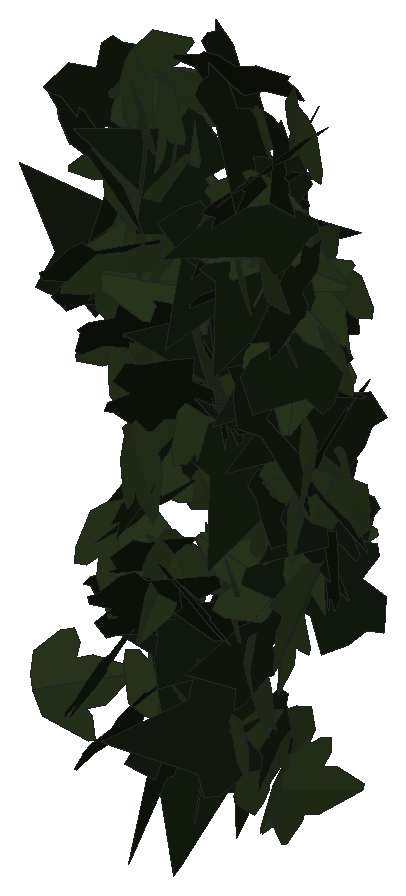
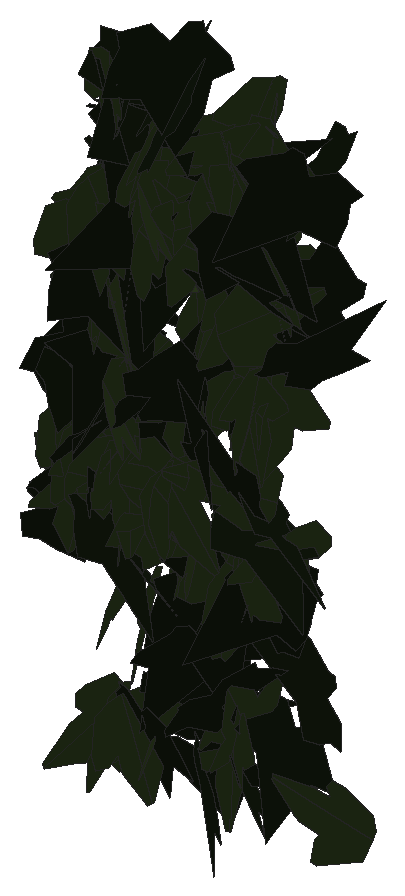
# SketchUp Ruby script. Lengths in inches.
U = 1.inch
M = Sketchup.active_model
def pt(a) = Geom::Point3d.new(a.map { |v| v * U })
def face(e, loops, mat)
  f = e.add_face(loops[0].map { |a| pt(a) })
  loops[1..].each { |l| e.add_face(l.map { |a| pt(a) }).erase! }
  f.material = f.back_material = mat if mat
  f
end
# faces: each face lists its corners as indices into pts; further lists are holes
def faces(e, pts, list, mat = nil) = list.each { |f| face(e, (f[0].is_a?(Array) ? f : [f]).map { |l| l.map { |i| pts[i] } }, mat) }
# xy, xz, yz: faces in a plane at the given z, y or x. An outline is a flat list of corners, or four numbers for a rectangle; further outlines are holes
def ring(l) = l.size == 4 ? [[l[0], l[1]], [l[2], l[1]], [l[2], l[3]], [l[0], l[3]]] : l.each_slice(2).to_a
def flat(e, list, mat, &to3) = list.each { |f| face(e, (f[0].is_a?(Array) ? f : [f]).map { |l| ring(l).map { |u, v| to3.(u, v) } }, mat) }
def xy(e, z, list, mat = nil) = flat(e, list, mat) { |x, y| [x, y, z] }
def xz(e, y, list, mat = nil) = flat(e, list, mat) { |x, z| [x, y, z] }
def yz(e, x, list, mat = nil) = flat(e, list, mat) { |y, z| [x, y, z] }
def lines(e, pts, list) = list.each { |a, b| e.add_line(pt(pts[a]), pt(pts[b])) }
# prism: a flat outline (further loops are holes) pulled along v
def prism(e, loops, v, mat = nil)
  f = face(e, loops, mat); d = Geom::Vector3d.new(v.map { |x| x * U })
  f.pushpull(f.normal.samedirection?(d) ? d.length : -d.length)
end
def box(e, o, s, mat = nil) = prism(e, [[o, [o[0] + s[0], o[1], o[2]], [o[0] + s[0], o[1] + s[1], o[2]], [o[0], o[1] + s[1], o[2]]]], [0, 0, s[2]], mat)
def at(x, y, z, deg = 0) = Geom::Transformation.translation(pt([x, y, z])) * Geom::Transformation.rotation(ORIGIN, Z_AXIS, deg.degrees)
def axes(o, x, y, z) = Geom::Transformation.new([*x, 0, *y, 0, *z, 0, *pt(o).to_a, 1])
def part(name) = M.definitions.add(name)
# library, detail: a bought-in or finely detailed component or shape, given as its bounding box
def library(name, o, s) = part(name).tap { |d| box(d.entities, o, s) }
def detail(e, o, s) = box(e.add_group.entities, o, s)
def put(e, d, t, mat = nil) = e.add_instance(d, t).tap { |i| i.material = mat if mat }
def group(e, t, mat = nil) = e.add_group.tap { |g| g.transformation = t; g.material = mat if mat }.entities
root = M.entities
M.materials.add("efeu1").color = [18, 25, 13]
M.materials.add("efeu2").color = [43, 57, 29]
c1 = part("ivyleaf_10")
p = [[0,0.5,-0.03],[-0.0625,2.02,-0.43],[-0.19,2.01,-0.46],[-0.54,1.05,-0.29],[-0.52,0.625,-0.18],[-0.83,0.76,-0.28],
  [-1.16,0.64,-0.33],[-1.15,0.33,-0.24],[-0.77,-0.39,0.02],[-0.3,-0.51,0.16],[0.04,-0.48,0.23],[-0.02,2.01,-0.4375],
  [-0.06,2.01,-0.43],[0.04,-0.49,0.23],[0.67,-0.49,0.14],[1.38,0.36,-0.2],[1.375,0.51,-0.24],[0.81,0.65,-0.19],
  [0.62,0.59,-0.15],[0.6,1.09,-0.28],[0.5,1.23,-0.31]]
faces(c1.entities,p,[[0,1,2,3,4,5,6,7,8,9,10],[11,12,0,13,14,15,16,17,18,19,20]],"efeu2")
c2 = part("ivyleaf_9")
p = [[1.54,2.16,1.25],[1.36,2.04,1.19],[-0.21,0.99,0.68],[-0.71,1.11,0.82],[-0.85,0.86,0.67],[-0.8,0.17,0.21],
  [-0.9,-0.01,0.1],[-0.67,-0.16,-0.02],[-0.08,-0.08,-0.05],[-0.03,-0.6,-0.4],[0.65,-0.88,-0.66],[0.83,-0.6,-0.49],
  [1.29,-0.42,-0.43],[1.8125,-0.07,-0.26],[1.21,0.44,0.15]]
faces(c2.entities,p,[[0,1,2,3,4,5,6,7,8,9,10,11,12,13,14]],"efeu1")
put(root,c1,axes([51.53,222.47,218.5625],[-0.09013,0.46947,0.14655],[-0.095,0.12957,-0.47348],[-0.48255,-0.11319,0.06584]))
put(root,c2,axes([50.85,222.37,215.3],[-0.1452,0.47845,-0.00029],[-0.00094,0.00002,0.5],[0.47845,0.1452,0.0009]))
put(root,c2,axes([51.6,222.35,219.3125],[0.35261,0.16273,0.31494],[0.29339,0.11538,-0.38809],[-0.19898,0.45848,-0.01412]))
put(root,c2,axes([53.29,222.89,221.95],[-0.4713,-0.01796,0.166],[-0.152,-0.15955,-0.44882],[0.06909,-0.47352,0.14493]))
put(root,c2,axes([53.6,222.66,221.11],[-0.40142,0.29572,0.03759],[-0.03003,0.02261,-0.49859],[-0.29659,-0.40254,-0.00039]))
put(root,c1,axes([53.06,222.78,221.97],[0.37689,0.10748,-0.31049],[-0.3067,-0.05441,-0.39112],[-0.11786,0.48527,0.02491]))
put(root,c1,axes([51.17,222.7,220.59],[-0.27641,-0.41637,-0.01513],[0.00782,0.01297,-0.49977],[0.41657,-0.27652,-0.00066]))
put(root,c2,axes([50.44,222.85,222.03],[0.31276,-0.37154,0.1189],[0.08783,-0.08142,-0.48544],[0.38009,0.32454,0.01433]))
put(root,c2,axes([53,222.84,222.1],[-0.1065,0.34539,-0.34549],[0.01072,-0.35187,-0.35507],[-0.48841,-0.08304,0.06754]))
put(root,c1,axes([51.28,222.55,220.52],[0.32321,-0.38109,-0.01756],[0.38148,0.32305,0.01069],[0.0032,-0.02031,0.49958]))
put(root,c2,axes([52.9,223.02,221.21],[-0.35666,-0.34673,-0.05072],[0.0462,0.02521,-0.49722],[0.34736,-0.35937,0.01405]))
put(root,c1,axes([51.41,222.7,222.22],[0.2972,-0.3609,-0.17726],[-0.02517,0.20329,-0.45611],[0.4013,0.28004,0.10267]))
put(root,c1,axes([51.01,222.82,217.28],[0.21033,0.447,-0.07716],[-0.03053,-0.0709,-0.494],[-0.45258,0.21252,-0.00253]))
put(root,c2,axes([51.21,222.53,216.45],[0.19094,0.36808,-0.27939],[0.12822,0.24824,0.41465],[0.44396,-0.22999,0.00041]))
put(root,c2,axes([50.56,222.55,220.26],[0.20508,0.39106,-0.23455],[0.09026,0.21728,0.44118],[0.44699,-0.22329,0.01853]))
put(root,c1,axes([53.11,222.69,221.28],[-0.39687,0.26741,0.14488],[-0.13605,0.05692,-0.47775],[-0.27201,-0.41863,0.02758]))
put(root,c1,axes([51.57,223.06,216.97],[0.04111,0.35247,-0.35225],[-0.05375,-0.34824,-0.35474],[-0.4954,0.06703,0.00926]))
put(root,c2,axes([52.31,223.21,222.66],[0.07999,-0.40668,0.27966],[0.05668,-0.27387,-0.41447],[0.4903,0.09801,0.00229]))
put(root,c1,axes([53.36,223.11,217.25],[0.11599,-0.43936,0.20859],[0.05478,-0.20127,-0.45441],[0.48326,0.12827,0.00144]))
put(root,c2,axes([52.375,223.15,215.03],[-0.2948,-0.08589,0.39461],[-0.37797,-0.11338,-0.30705],[0.14223,-0.47934,0.00192]))
put(root,c2,axes([51.16,222.59,219.98],[0.24192,0.42964,0.083],[0.04242,0.07137,-0.49306],[-0.43552,0.2456,-0.00191]))
put(root,c2,axes([52.2,223.27,221.01],[-0.19816,-0.42517,0.1731],[-0.07988,-0.15373,-0.46903],[0.45205,-0.21354,-0.007]))
put(root,c1,axes([51.1,222.91,221.77],[-0.42511,-0.26303,0.00996],[-0.00843,-0.00531,-0.4999],[0.26309,-0.42519,0.00008]))
put(root,c2,axes([51.81,223.1875,221.69],[-0.2757,-0.30734,-0.28201],[-0.07306,-0.29724,0.39536],[-0.41067,0.25921,0.11899]))
put(root,c2,axes([51.08,222.61,214.89],[0.04356,0.45929,0.19275],[-0.00147,0.1936,-0.46099],[-0.4981,0.03959,0.01822]))
put(root,c2,axes([52.98,222.91,216.44],[-0.38657,0.28802,0.1327],[-0.11215,0.07154,-0.48198],[-0.29662,-0.4024,0.00929]))
put(root,c2,axes([51.43,223.17,214.69],[-0.33422,0.06395,-0.36634],[0.34404,-0.13384,-0.33723],[-0.14119,-0.47749,0.04546]))
put(root,c1,axes([50.98,223.07,220.77],[0.40347,-0.29013,0.05512],[0.05387,-0.01946,-0.49671],[0.29037,0.40675,0.01556]))
put(root,c2,axes([51.63,222.87,216.83],[0.48565,-0.10855,-0.04857],[-0.04435,0.02414,-0.49744],[0.11034,0.48748,0.01382]))
put(root,c2,axes([53.11,222.68,222.45],[0.02571,0.48637,0.11306],[-0.06647,0.11554,-0.48191],[-0.49489,0.00975,0.0706]))
put(root,c1,axes([52.13,222.86,219.76],[-0.39035,0.30083,0.08443],[-0.06397,0.05529,-0.4928],[-0.30583,-0.39553,-0.00468]))
put(root,c2,axes([52.76,223.12,219.43],[0.23713,-0.43991,-0.01563],[-0.00319,0.01603,-0.49973],[0.44018,0.23711,0.00479]))
put(root,c1,axes([51.18,222.89,222.6],[-0.35461,0.33294,0.11578],[-0.11976,0.04067,-0.48374],[-0.33153,-0.3708,0.0509]))
put(root,c1,axes([51.25,223.08,222.47],[0.48012,-0.1225,0.06694],[0.06603,-0.01194,-0.49548],[0.12299,0.48461,0.00472]))
put(root,c2,axes([51.3125,222.97,217.94],[-0.3635,0.34265,-0.0214],[0.00742,-0.02331,-0.4994],[-0.34324,-0.36338,0.01186]))
put(root,c2,axes([52.96,223.37,222.04],[-0.0399,-0.16713,0.46955],[0.04881,-0.4701,-0.16318],[0.49601,0.03282,0.05383]))
put(root,c1,axes([53.45,222.97,218.9375],[0.307,-0.34197,-0.19701],[-0.12092,0.15609,-0.45936],[0.37568,0.32969,0.01314]))
put(root,c2,axes([52.61,223.28,218.59],[-0.32666,-0.37805,-0.01928],[0.02806,0.00121,-0.49921],[0.3775,-0.32723,0.02043]))
put(root,c1,axes([52.89,222.79,216.09],[-0.25643,0.34097,0.26074],[-0.16356,0.20319,-0.42657],[-0.39685,-0.30406,0.00733]))
put(root,c1,axes([52.74,222.79,221.16],[-0.19654,0.2832,0.36217],[-0.25024,0.26453,-0.34265],[-0.38569,-0.31594,0.03776]))
put(root,c2,axes([51.11,222.72,216.8125],[0.32163,0.31644,0.21546],[0.15633,0.14831,-0.45118],[-0.34945,0.35759,-0.00354]))
put(root,c2,axes([53.35,223.28,220.15],[-0.47332,-0.13365,0.09004],[-0.08956,-0.0141,-0.49171],[0.13398,-0.4816,-0.0106]))
put(root,c1,axes([52.08,223.02,218.92],[0.15085,0.47494,0.04094],[0.01149,0.0393,-0.49832],[-0.47656,0.15129,0.00094]))
put(root,c2,axes([51.79,223.27,214.66],[-0.36635,-0.2752,-0.20014],[0.17887,0.09443,-0.45726],[0.28947,-0.40663,0.02926]))
put(root,c1,axes([52.68,223.29,216.9375],[0.03155,0.37974,0.32373],[-0.13343,-0.30614,0.37212],[0.48084,-0.10987,0.08202]))
put(root,c2,axes([51.3,222.93,217.53],[-0.10984,0.48344,0.06497],[-0.17872,0.02208,-0.46645],[-0.45387,-0.12569,0.16795]))
put(root,c2,axes([52.46,222.82,220.73],[0.12701,0.47411,0.09533],[0.02348,0.0924,-0.49083],[-0.48303,0.12916,0.0012]))
put(root,c1,axes([52.88,222.89,221.27],[0.12881,0.12552,0.46653],[0.29401,0.36276,-0.17878],[-0.38336,0.32039,0.01965]))
put(root,c1,axes([51.62,223.32,221.64],[0.01238,-0.47706,0.14921],[0.00876,-0.14903,-0.47719],[0.49977,0.01442,0.00467]))
put(root,c1,axes([52.09,223.14,217.17],[-0.35056,0.33673,-0.11712],[0.07896,-0.08685,-0.48603],[-0.34767,-0.35926,0.00771]))
put(root,c1,axes([53.17,223.21,220.09],[0.47323,0.16101,-0.0113],[-0.00985,-0.00615,-0.49987],[-0.1611,0.47333,-0.00265]))
put(root,c2,axes([51.93,223.05,216.51],[0.19764,0.30189,-0.34612],[-0.31667,-0.18334,-0.34074],[-0.33265,0.3539,0.11873]))
put(root,c1,axes([51.48,223.17,216.875],[-0.49501,-0.06741,-0.02064],[0.0255,-0.0347,-0.49814],[0.06572,-0.49422,0.03779]))
put(root,c1,axes([51.17,223.03,222.89],[0.00027,0.46119,0.19313],[-0.04802,0.19226,-0.45905],[-0.49769,-0.0183,0.04439]))
put(root,c1,axes([51.14,223.3,221.14],[0.46198,-0.19074,0.01372],[0.01541,0.00136,-0.49976],[0.19061,0.46219,0.00713]))
put(root,c2,axes([53.43,223.55,219.4],[-0.02353,-0.00215,-0.49944],[-0.01571,-0.49974,0.00289],[-0.4992,0.01583,0.02345]))
put(root,c1,axes([51.24,223.35,222.01],[0.38231,-0.30441,0.10571],[0.09256,-0.05338,-0.48845],[0.30866,0.39305,0.01554]))
put(root,c1,axes([52.47,223.35,214.46],[-0.24668,0.39786,0.17567],[0.08856,-0.15178,0.4681],[0.4258,0.26205,0.00442]))
put(root,c1,axes([50.93,223.23,219.35],[-0.39797,-0.29994,-0.04077],[0.04729,0.00491,-0.49773],[0.29898,-0.40002,0.02446]))
put(root,c1,axes([52.52,223.24,219.33],[-0.39228,-0.09134,-0.29626],[0.30715,-0.0496,-0.39141],[0.04211,-0.48908,0.09502]))
put(root,c1,axes([52.96,223.07,220.53],[-0.3315,0.27457,0.25441],[-0.1984,0.15929,-0.43042],[-0.31741,-0.38632,0.00334]))
put(root,c1,axes([51.69,223.51,221.04],[0.12761,0.30354,-0.37627],[-0.18856,-0.32708,-0.32781],[-0.44515,0.22557,0.03099]))
put(root,c1,axes([53.18,223.05,220.83],[0.19108,0.34581,0.30643],[0.13762,0.27396,-0.39498],[-0.44108,0.23529,0.00952]))
put(root,c1,axes([50.98,223.62,220.36],[0.03595,0.11443,0.4854],[-0.08897,-0.47738,0.11913],[0.49071,-0.09494,-0.01396]))
put(root,c1,axes([53.41,223.39,218.3],[-0.33555,-0.32518,0.17795],[-0.11686,-0.13499,-0.46703],[0.35178,-0.35501,0.01459]))
put(root,c1,axes([51.25,223.37,222.12],[0.48185,-0.13169,0.02194],[0.02064,-0.00771,-0.49951],[0.1319,0.48229,-0.00199]))
put(root,c2,axes([52.86,223.26,218.21],[0.31517,-0.34938,-0.16912],[-0.07936,0.15525,-0.46861],[0.37996,0.32223,0.0424]))
put(root,c1,axes([51,222.98,218.82],[-0.03076,0.30846,-0.39231],[-0.04672,0.38955,0.30995],[0.49686,0.05573,0.00486]))
put(root,c1,axes([52.03,223.61,217.88],[0.05642,-0.37226,0.329],[0.14289,-0.30497,-0.36956],[0.47581,0.13572,0.07197]))
put(root,c1,axes([53.07,223.49,221.17],[-0.09679,-0.4682,0.14635],[-0.02115,-0.14505,-0.47803],[0.49009,-0.09872,0.00827]))
put(root,c1,axes([52.75,223.34,217.92],[-0.14419,-0.47616,-0.04978],[0.02198,0.04535,-0.49745],[0.47825,-0.14564,0.00786]))
put(root,c1,axes([52.84,223.64,214.71],[0.01119,0.25748,-0.42846],[-0.02079,-0.42796,-0.25772],[-0.49944,0.02358,0.00113]))
put(root,c1,axes([52.75,223.59,216.55],[-0.08412,0.30386,-0.38807],[0.09433,-0.37647,-0.31523],[-0.48376,-0.12625,0.00601]))
put(root,c1,axes([51.08,223.41,220.3125],[0.15514,0.44937,-0.15492],[-0.13336,-0.11527,-0.4679],[-0.45623,0.1865,0.08409]))
put(root,c1,axes([52.09,223.4,221.05],[0.26089,0.10886,0.41241],[-0.38726,-0.14218,0.28251],[0.17879,-0.46683,0.01013]))
put(root,c1,axes([53.36,223.33,220.13],[-0.45889,0.16917,0.10395],[-0.12408,-0.03996,-0.48271],[-0.15501,-0.46881,0.07866]))
put(root,c1,axes([51.46,223.49,220.67],[0.38,-0.14036,0.29308],[0.28475,-0.07344,-0.40438],[0.15657,0.47424,0.02412]))
put(root,c1,axes([51.15,223.19,218.05],[-0.08021,-0.06175,0.48964],[0.38399,0.30381,0.10122],[-0.31002,0.39228,-0.00131]))
put(root,c2,axes([50.36,223.5,220.02],[-0.27996,-0.41241,-0.03924],[-0.01347,-0.03827,0.49835],[-0.41406,0.28009,0.01032]))
put(root,c2,axes([53.65,223.6,217.19],[-0.14846,-0.2032,-0.43205],[-0.26405,-0.34202,0.25159],[-0.39779,0.30287,-0.00576]))
put(root,c1,axes([53.04,223.56,218.45],[0.19591,0.36789,-0.27618],[-0.12846,-0.24449,-0.4168],[-0.44172,0.23426,-0.00128]))
put(root,c2,axes([52.99,223.13,219.34],[0.2937,0.4046,-0.00625],[-0.00348,-0.00519,-0.49996],[-0.40463,0.29372,-0.00023]))
put(root,c2,axes([52,223.21,219.11],[0.08115,0.02919,-0.49251],[-0.49185,0.04398,-0.07843],[0.03875,0.49721,0.03585]))
put(root,c2,axes([52.29,223.22,223.2],[0.18846,0.37484,-0.27199],[-0.30327,-0.12204,-0.37833],[-0.35001,0.30757,0.18136]))
put(root,c1,axes([51.24,223.37,222.53],[-0.45165,-0.21393,-0.01567],[0.01291,0.00935,-0.49975],[0.21411,-0.45183,-0.00292]))
put(root,c1,axes([53.05,223.39,222.67],[-0.40635,0.27842,0.08581],[-0.14658,-0.0681,-0.47316],[-0.25179,-0.40969,0.13696]))
put(root,c1,axes([51.27,223.13,215.12],[0.06966,0.38882,-0.30654],[0.00813,0.30862,0.3933],[0.49506,-0.05979,0.03667]))
put(root,c1,axes([52.35,223.33,221.69],[-0.15928,-0.44128,-0.17291],[0.05543,0.16382,-0.46914],[0.4707,-0.16862,-0.00327]))
put(root,c2,axes([52.97,223.02,221.98],[0.06667,0.20547,0.45093],[0.02258,0.45326,-0.20987],[-0.49502,0.04835,0.05116]))
put(root,c1,axes([51.31,223.48,222.44],[0.34625,0.34729,-0.09746],[-0.07392,-0.06391,-0.49036],[-0.35305,0.35399,0.00709]))
put(root,c2,axes([53.02,223.42,220.42],[0.06208,0.38261,-0.31584],[-0.08304,-0.3058,-0.38677],[-0.48913,0.10048,0.02558]))
put(root,c2,axes([51.02,223.58,221.64],[-0.05127,0.28914,-0.40468],[0.02246,-0.40507,-0.29226],[-0.49686,-0.04815,0.02855]))
put(root,c1,axes([53.12,223.64,218.13],[0.16383,0.32602,-0.34187],[-0.20669,-0.2759,-0.36216],[-0.42478,0.25999,0.04437]))
put(root,c1,axes([53.18,223.12,214.66],[-0.07641,-0.18223,-0.4593],[0.18234,0.42156,-0.19759],[0.45925,-0.19769,0.00203]))
put(root,c2,axes([51.33,223.66,220.86],[-0.49277,-0.07513,0.0391],[-0.02874,-0.06878,-0.49441],[0.07967,-0.48951,0.06346]))
put(root,c2,axes([51.85,223.19,214.4],[-0.08984,0.03047,-0.49092],[-0.46284,0.16366,0.09486],[0.16646,0.47147,-0.0012]))
put(root,c1,axes([53.03,223.65,217.85],[0.14909,0.05549,-0.47402],[-0.43084,-0.19797,-0.15869],[-0.20529,0.45577,-0.01122]))
put(root,c1,axes([51.38,223.34,215.05],[-0.42936,0.16469,0.19629],[-0.18586,0.0635,-0.45981],[-0.17638,-0.46781,0.00669]))
put(root,c2,axes([51.74,223.41,216.11],[-0.00967,-0.3585,-0.3484],[0.03444,0.34716,-0.35818],[0.49872,-0.03093,0.01798]))
put(root,c1,axes([49.625,223.4375,214.56],[0.17987,-0.03035,-0.46554],[0.46542,-0.02266,0.1813],[-0.0321,-0.49856,0.02009]))
put(root,c1,axes([51.15,223.45,219.41],[-0.44825,-0.02206,0.22041],[-0.21933,-0.02558,-0.4486],[0.03107,-0.49886,0.01325]))
put(root,c2,axes([51.35,223.4,218.18],[-0.31461,0.24156,0.30441],[0.21795,-0.21459,0.39554],[0.32174,0.38158,0.02973]))
put(root,c1,axes([52.1,223.79,221.12],[-0.02006,-0.35152,0.35501],[0.1703,-0.33883,-0.32587],[0.46968,0.10784,0.13332]))
put(root,c1,axes([53.2,223.36,218.07],[-0.01554,0.48945,0.10096],[-0.06358,0.09826,-0.48611],[-0.4957,-0.02795,0.05919]))
put(root,c1,axes([51.01,223.34,219.51],[-0.11925,0.46578,0.13723],[-0.07676,0.12145,-0.47891],[-0.47946,-0.13529,0.04254]))
put(root,c2,axes([53.27,223.91,218.03],[-0.20558,-0.32747,0.31702],[-0.1331,-0.28948,-0.38533],[0.43591,-0.24282,0.03185]))
put(root,c2,axes([53.46,223.61,219.11],[-0.28828,0.29453,-0.2831],[0.19016,-0.20992,-0.41203],[-0.36157,-0.34523,0.00902]))
put(root,c2,axes([51.24,223.78,215.79],[-0.12178,-0.48465,0.01693],[-0.00567,-0.01603,-0.49971],[0.48491,-0.12191,-0.00159]))
put(root,c2,axes([52.99,223.47,218.75],[0.34613,-0.31741,-0.17159],[-0.11311,0.13033,-0.46927],[0.34263,0.36368,0.01842]))
put(root,c1,axes([52.65,223.73,218.97],[0.21128,-0.39674,0.21899],[0.1089,-0.19009,-0.44945],[0.43989,0.23762,0.00609]))
put(root,c1,axes([53.24,223.45,217.64],[0.12375,0.48126,0.05548],[0.0215,0.05175,-0.49685],[-0.48397,0.12535,-0.00788]))
put(root,c1,axes([52.54,223.62,214.99],[-0.17445,-0.45888,0.09483],[-0.03714,-0.08733,-0.49091],[0.46711,-0.17832,-0.00362]))
put(root,c2,axes([52.3,223.67,215.13],[-0.39072,-0.0338,-0.31015],[0.30854,0.03184,-0.39216],[0.04626,-0.49784,-0.00402]))
put(root,c2,axes([53.49,223.32,217.15],[0.05235,-0.09557,0.48798],[-0.12742,0.47172,0.10605],[-0.48065,-0.13546,0.02503]))
put(root,c2,axes([53.01,223.43,217.25],[-0.23202,0.44157,-0.03431],[0.00573,-0.03574,-0.49869],[-0.44287,-0.23181,0.01152]))
put(root,c1,axes([52.05,223.53,217.92],[-0.31355,-0.02267,0.38881],[-0.38669,-0.04144,-0.31425],[0.04647,-0.49776,0.00845]))
put(root,c1,axes([53.26,223.57,220.83],[-0.48481,-0.05901,0.10715],[-0.0968,-0.08271,-0.48352],[0.07478,-0.48957,0.06877]))
put(root,c1,axes([52.36,223.48,222.19],[-0.23331,0.44164,0.02282],[-0.00835,0.0214,-0.49947],[-0.44215,-0.23344,-0.00261]))
put(root,c1,axes([52.65,223.65,220.02],[0.2612,-0.42635,-0.00123],[-0.00062,0.00106,-0.5],[0.42635,0.2612,0.00003]))
put(root,c2,axes([51.77,223.9375,222.625],[0.05624,-0.3425,0.3599],[0.07906,-0.35142,-0.34678],[0.4905,0.09591,0.01463]))
put(root,c2,axes([50.26,223.42,222.35],[-0.04873,-0.14106,-0.47721],[0.15199,0.45236,-0.14923],[0.47384,-0.15961,-0.0012]))
put(root,c1,axes([52.11,223.8,221.64],[0.2245,-0.40532,0.18793],[0.09673,-0.16123,-0.4633],[0.43617,0.24437,0.00602]))
put(root,c2,axes([52.3,223.64,218.95],[-0.19443,-0.42966,0.1661],[0.06703,0.15198,0.4716],[-0.45575,0.20565,-0.0015]))
put(root,c1,axes([53.22,223.66,217.86],[-0.48108,-0.05273,0.12561],[0.1248,0.01429,0.48396],[-0.05463,0.49701,-0.00058]))
put(root,c2,axes([51.94,223.9,219.32],[-0.1968,-0.04344,0.45758],[-0.40577,-0.21741,-0.19516],[0.21592,-0.44816,0.05032]))
put(root,c2,axes([52.33,223.26,221.11],[0.29112,0.23669,0.33049],[0.25847,0.20597,-0.37519],[-0.31375,0.3893,-0.00243]))
